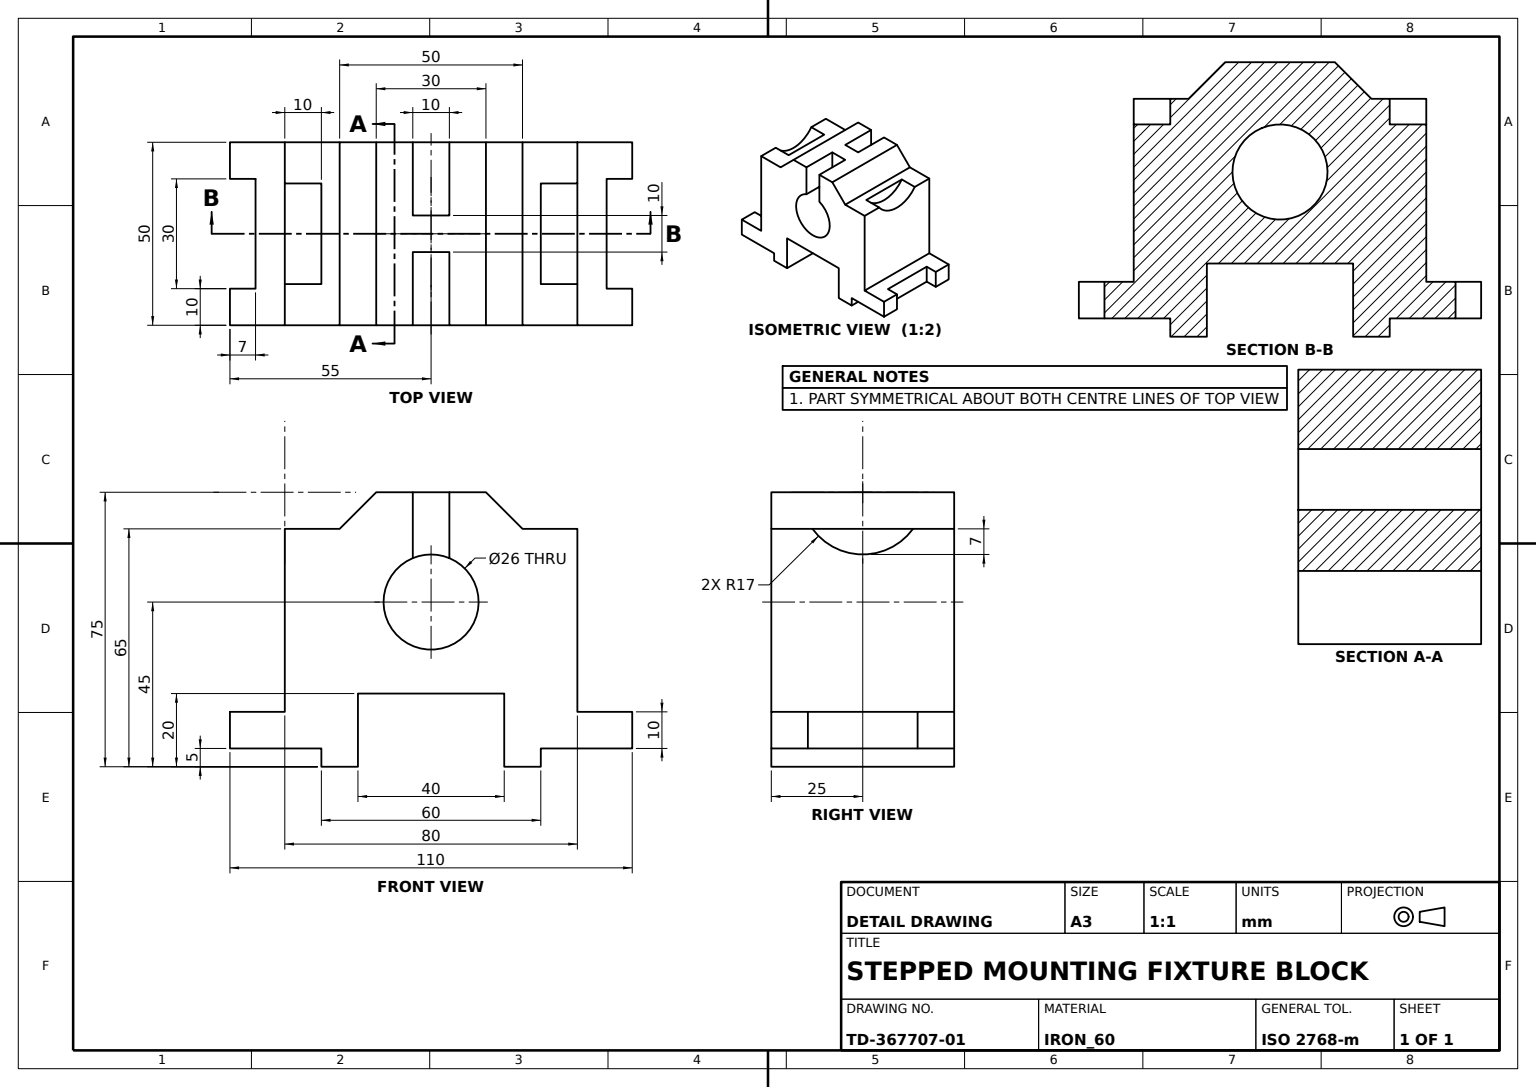
ISO-10303-21;
HEADER;
FILE_DESCRIPTION((''),'2;1');
FILE_NAME('','',(''),(''),'','','');
FILE_SCHEMA(('AUTOMOTIVE_DESIGN'));
ENDSEC;
DATA;
#1=APPLICATION_CONTEXT('');
#2=PRODUCT_CONTEXT('',#1,'mechanical');
#3=PRODUCT('','','',(#2));
#4=PRODUCT_DEFINITION_FORMATION('','',#3);
#5=PRODUCT_DEFINITION_CONTEXT('',#1,'design');
#6=PRODUCT_DEFINITION('','',#4,#5);
#7=PRODUCT_DEFINITION_SHAPE('','',#6);
#8=(LENGTH_UNIT()NAMED_UNIT(*)SI_UNIT(.MILLI.,.METRE.));
#9=(NAMED_UNIT(*)PLANE_ANGLE_UNIT()SI_UNIT($,.RADIAN.));
#10=(NAMED_UNIT(*)SI_UNIT($,.STERADIAN.)SOLID_ANGLE_UNIT());
#11=UNCERTAINTY_MEASURE_WITH_UNIT(LENGTH_MEASURE(0.005),#8,'distance_accuracy_value','');
#12=(GEOMETRIC_REPRESENTATION_CONTEXT(3)GLOBAL_UNCERTAINTY_ASSIGNED_CONTEXT((#11))GLOBAL_UNIT_ASSIGNED_CONTEXT((#8,#9,#10))REPRESENTATION_CONTEXT('',''));
#13=CARTESIAN_POINT('',(13.747727,-30.,60.));
#14=VERTEX_POINT('',#13);
#15=CARTESIAN_POINT('',(-13.747727,-30.,60.));
#16=VERTEX_POINT('',#15);
#17=CARTESIAN_POINT('',(25.,-30.,60.));
#18=DIRECTION('',(-1.,0.,0.));
#19=VECTOR('',#18,1000.);
#20=LINE('',#17,#19);
#21=EDGE_CURVE('',#14,#16,#20,.T.);
#22=ORIENTED_EDGE('',*,*,#21,.T.);
#23=CARTESIAN_POINT('',(0.,-30.,70.));
#24=DIRECTION('',(0.,-1.,0.));
#25=DIRECTION('',(1.,0.,0.));
#26=AXIS2_PLACEMENT_3D('',#23,#24,#25);
#27=CIRCLE('',#26,17.);
#28=EDGE_CURVE('',#14,#16,#27,.F.);
#29=ORIENTED_EDGE('',*,*,#28,.F.);
#30=EDGE_LOOP('',(#22,#29));
#31=FACE_BOUND('',#30,.T.);
#32=DIRECTION('',(0.,0.,-1.));
#33=AXIS2_PLACEMENT_3D('',#23,#24,#32);
#34=PLANE('',#33);
#35=ADVANCED_FACE('',(#31),#34,.T.);
#36=CARTESIAN_POINT('',(-15.,-55.,10.));
#37=VERTEX_POINT('',#36);
#38=CARTESIAN_POINT('',(-15.,-48.,10.));
#39=VERTEX_POINT('',#38);
#40=DIRECTION('',(0.,1.,0.));
#41=VECTOR('',#40,1000.);
#42=LINE('',#36,#41);
#43=EDGE_CURVE('',#37,#39,#42,.T.);
#44=ORIENTED_EDGE('',*,*,#43,.T.);
#45=CARTESIAN_POINT('',(15.,-48.,10.));
#46=VERTEX_POINT('',#45);
#47=CARTESIAN_POINT('',(25.,-48.,10.));
#48=VECTOR('',#25,1000.);
#49=LINE('',#47,#48);
#50=EDGE_CURVE('',#39,#46,#49,.T.);
#51=ORIENTED_EDGE('',*,*,#50,.T.);
#52=CARTESIAN_POINT('',(15.,-55.,10.));
#53=VERTEX_POINT('',#52);
#54=VECTOR('',#24,1000.);
#55=LINE('',#52,#54);
#56=EDGE_CURVE('',#46,#53,#55,.T.);
#57=ORIENTED_EDGE('',*,*,#56,.T.);
#58=CARTESIAN_POINT('',(25.,-55.,10.));
#59=VERTEX_POINT('',#58);
#60=LINE('',#58,#19);
#61=EDGE_CURVE('',#59,#53,#60,.T.);
#62=ORIENTED_EDGE('',*,*,#61,.F.);
#63=CARTESIAN_POINT('',(25.,-40.,10.));
#64=VERTEX_POINT('',#63);
#65=LINE('',#58,#41);
#66=EDGE_CURVE('',#59,#64,#65,.T.);
#67=ORIENTED_EDGE('',*,*,#66,.T.);
#68=CARTESIAN_POINT('',(-25.,-40.,10.));
#69=VERTEX_POINT('',#68);
#70=LINE('',#63,#19);
#71=EDGE_CURVE('',#64,#69,#70,.T.);
#72=ORIENTED_EDGE('',*,*,#71,.T.);
#73=CARTESIAN_POINT('',(-25.,-55.,10.));
#74=VERTEX_POINT('',#73);
#75=LINE('',#73,#41);
#76=EDGE_CURVE('',#74,#69,#75,.T.);
#77=ORIENTED_EDGE('',*,*,#76,.F.);
#78=EDGE_CURVE('',#37,#74,#60,.T.);
#79=ORIENTED_EDGE('',*,*,#78,.F.);
#80=EDGE_LOOP('',(#44,#51,#57,#62,#67,#72,#77,#79));
#81=FACE_BOUND('',#80,.T.);
#82=DIRECTION('',(0.,0.,1.));
#83=AXIS2_PLACEMENT_3D('',#58,#82,#25);
#84=PLANE('',#83);
#85=ADVANCED_FACE('',(#81),#84,.T.);
#86=CARTESIAN_POINT('',(25.,-40.,60.));
#87=VERTEX_POINT('',#86);
#88=CARTESIAN_POINT('',(13.747727,-40.,60.));
#89=VERTEX_POINT('',#88);
#90=LINE('',#86,#19);
#91=EDGE_CURVE('',#87,#89,#90,.T.);
#92=ORIENTED_EDGE('',*,*,#91,.F.);
#93=CARTESIAN_POINT('',(25.,-25.,60.));
#94=VERTEX_POINT('',#93);
#95=CARTESIAN_POINT('',(25.,40.,60.));
#96=LINE('',#95,#54);
#97=EDGE_CURVE('',#94,#87,#96,.T.);
#98=ORIENTED_EDGE('',*,*,#97,.F.);
#99=CARTESIAN_POINT('',(-25.,-25.,60.));
#100=VERTEX_POINT('',#99);
#101=LINE('',#93,#19);
#102=EDGE_CURVE('',#94,#100,#101,.T.);
#103=ORIENTED_EDGE('',*,*,#102,.T.);
#104=CARTESIAN_POINT('',(-25.,-40.,60.));
#105=VERTEX_POINT('',#104);
#106=CARTESIAN_POINT('',(-25.,40.,60.));
#107=LINE('',#106,#54);
#108=EDGE_CURVE('',#100,#105,#107,.T.);
#109=ORIENTED_EDGE('',*,*,#108,.T.);
#110=CARTESIAN_POINT('',(-13.747727,-40.,60.));
#111=VERTEX_POINT('',#110);
#112=EDGE_CURVE('',#111,#105,#90,.T.);
#113=ORIENTED_EDGE('',*,*,#112,.F.);
#114=CARTESIAN_POINT('',(-13.747727,-45.,60.));
#115=LINE('',#114,#41);
#116=EDGE_CURVE('',#16,#111,#115,.F.);
#117=ORIENTED_EDGE('',*,*,#116,.F.);
#118=ORIENTED_EDGE('',*,*,#21,.F.);
#119=CARTESIAN_POINT('',(13.747727,-45.,60.));
#120=LINE('',#119,#41);
#121=EDGE_CURVE('',#89,#14,#120,.T.);
#122=ORIENTED_EDGE('',*,*,#121,.F.);
#123=EDGE_LOOP('',(#92,#98,#103,#109,#113,#117,#118,#122));
#124=FACE_BOUND('',#123,.T.);
#125=AXIS2_PLACEMENT_3D('',#95,#32,#18);
#126=PLANE('',#125);
#127=ADVANCED_FACE('',(#124),#126,.F.);
#128=CARTESIAN_POINT('',(25.,5.,70.));
#129=VERTEX_POINT('',#128);
#130=CARTESIAN_POINT('',(5.,5.,70.));
#131=VERTEX_POINT('',#130);
#132=LINE('',#128,#19);
#133=EDGE_CURVE('',#129,#131,#132,.T.);
#134=ORIENTED_EDGE('',*,*,#133,.F.);
#135=CARTESIAN_POINT('',(25.,15.,70.));
#136=VERTEX_POINT('',#135);
#137=LINE('',#135,#54);
#138=EDGE_CURVE('',#136,#129,#137,.T.);
#139=ORIENTED_EDGE('',*,*,#138,.F.);
#140=CARTESIAN_POINT('',(-25.,15.,70.));
#141=VERTEX_POINT('',#140);
#142=LINE('',#135,#19);
#143=EDGE_CURVE('',#136,#141,#142,.T.);
#144=ORIENTED_EDGE('',*,*,#143,.T.);
#145=CARTESIAN_POINT('',(-25.,5.,70.));
#146=VERTEX_POINT('',#145);
#147=LINE('',#140,#54);
#148=EDGE_CURVE('',#141,#146,#147,.T.);
#149=ORIENTED_EDGE('',*,*,#148,.T.);
#150=CARTESIAN_POINT('',(-5.,5.,70.));
#151=VERTEX_POINT('',#150);
#152=LINE('',#128,#48);
#153=EDGE_CURVE('',#146,#151,#152,.T.);
#154=ORIENTED_EDGE('',*,*,#153,.T.);
#155=CARTESIAN_POINT('',(-5.,-5.,70.));
#156=VERTEX_POINT('',#155);
#157=CARTESIAN_POINT('',(-5.,15.,70.));
#158=LINE('',#157,#54);
#159=EDGE_CURVE('',#151,#156,#158,.T.);
#160=ORIENTED_EDGE('',*,*,#159,.T.);
#161=CARTESIAN_POINT('',(-25.,-5.,70.));
#162=VERTEX_POINT('',#161);
#163=CARTESIAN_POINT('',(25.,-5.,70.));
#164=LINE('',#163,#19);
#165=EDGE_CURVE('',#156,#162,#164,.T.);
#166=ORIENTED_EDGE('',*,*,#165,.T.);
#167=CARTESIAN_POINT('',(-25.,-15.,70.));
#168=VERTEX_POINT('',#167);
#169=EDGE_CURVE('',#162,#168,#147,.T.);
#170=ORIENTED_EDGE('',*,*,#169,.T.);
#171=CARTESIAN_POINT('',(25.,-15.,70.));
#172=VERTEX_POINT('',#171);
#173=LINE('',#171,#19);
#174=EDGE_CURVE('',#172,#168,#173,.T.);
#175=ORIENTED_EDGE('',*,*,#174,.F.);
#176=VERTEX_POINT('',#163);
#177=EDGE_CURVE('',#176,#172,#137,.T.);
#178=ORIENTED_EDGE('',*,*,#177,.F.);
#179=CARTESIAN_POINT('',(5.,-5.,70.));
#180=VERTEX_POINT('',#179);
#181=LINE('',#163,#48);
#182=EDGE_CURVE('',#180,#176,#181,.T.);
#183=ORIENTED_EDGE('',*,*,#182,.F.);
#184=CARTESIAN_POINT('',(5.,15.,70.));
#185=LINE('',#184,#54);
#186=EDGE_CURVE('',#131,#180,#185,.T.);
#187=ORIENTED_EDGE('',*,*,#186,.F.);
#188=EDGE_LOOP('',(#134,#139,#144,#149,#154,#160,#166,#170,#175,#178,#183,#187));
#189=FACE_BOUND('',#188,.T.);
#190=AXIS2_PLACEMENT_3D('',#135,#32,#18);
#191=PLANE('',#190);
#192=ADVANCED_FACE('',(#189),#191,.F.);
#193=CARTESIAN_POINT('',(25.,-55.,0.));
#194=VERTEX_POINT('',#193);
#195=CARTESIAN_POINT('',(15.,-55.,0.));
#196=VERTEX_POINT('',#195);
#197=LINE('',#193,#19);
#198=EDGE_CURVE('',#194,#196,#197,.T.);
#199=ORIENTED_EDGE('',*,*,#198,.T.);
#200=CARTESIAN_POINT('',(15.,-48.,0.));
#201=VERTEX_POINT('',#200);
#202=CARTESIAN_POINT('',(15.,55.,0.));
#203=LINE('',#202,#41);
#204=EDGE_CURVE('',#196,#201,#203,.T.);
#205=ORIENTED_EDGE('',*,*,#204,.T.);
#206=CARTESIAN_POINT('',(-15.,-48.,0.));
#207=VERTEX_POINT('',#206);
#208=CARTESIAN_POINT('',(25.,-48.,0.));
#209=LINE('',#208,#19);
#210=EDGE_CURVE('',#201,#207,#209,.T.);
#211=ORIENTED_EDGE('',*,*,#210,.T.);
#212=CARTESIAN_POINT('',(-15.,-55.,0.));
#213=VERTEX_POINT('',#212);
#214=CARTESIAN_POINT('',(-15.,55.,0.));
#215=LINE('',#214,#54);
#216=EDGE_CURVE('',#207,#213,#215,.T.);
#217=ORIENTED_EDGE('',*,*,#216,.T.);
#218=CARTESIAN_POINT('',(-25.,-55.,0.));
#219=VERTEX_POINT('',#218);
#220=EDGE_CURVE('',#213,#219,#197,.T.);
#221=ORIENTED_EDGE('',*,*,#220,.T.);
#222=CARTESIAN_POINT('',(-25.,-30.,0.));
#223=VERTEX_POINT('',#222);
#224=CARTESIAN_POINT('',(-25.,55.,0.));
#225=LINE('',#224,#54);
#226=EDGE_CURVE('',#223,#219,#225,.T.);
#227=ORIENTED_EDGE('',*,*,#226,.F.);
#228=CARTESIAN_POINT('',(25.,-30.,0.));
#229=VERTEX_POINT('',#228);
#230=LINE('',#228,#19);
#231=EDGE_CURVE('',#229,#223,#230,.T.);
#232=ORIENTED_EDGE('',*,*,#231,.F.);
#233=CARTESIAN_POINT('',(25.,55.,0.));
#234=LINE('',#233,#54);
#235=EDGE_CURVE('',#229,#194,#234,.T.);
#236=ORIENTED_EDGE('',*,*,#235,.T.);
#237=EDGE_LOOP('',(#199,#205,#211,#217,#221,#227,#232,#236));
#238=FACE_BOUND('',#237,.T.);
#239=AXIS2_PLACEMENT_3D('',#233,#32,#18);
#240=PLANE('',#239);
#241=ADVANCED_FACE('',(#238),#240,.T.);
#242=ORIENTED_EDGE('',*,*,#71,.F.);
#243=VECTOR('',#32,1000.);
#244=LINE('',#86,#243);
#245=EDGE_CURVE('',#87,#64,#244,.T.);
#246=ORIENTED_EDGE('',*,*,#245,.F.);
#247=ORIENTED_EDGE('',*,*,#91,.T.);
#248=CARTESIAN_POINT('',(0.,-40.,70.));
#249=AXIS2_PLACEMENT_3D('',#248,#40,#82);
#250=CIRCLE('',#249,17.);
#251=EDGE_CURVE('',#111,#89,#250,.F.);
#252=ORIENTED_EDGE('',*,*,#251,.F.);
#253=ORIENTED_EDGE('',*,*,#112,.T.);
#254=LINE('',#104,#243);
#255=EDGE_CURVE('',#105,#69,#254,.T.);
#256=ORIENTED_EDGE('',*,*,#255,.T.);
#257=EDGE_LOOP('',(#242,#246,#247,#252,#253,#256));
#258=FACE_BOUND('',#257,.T.);
#259=AXIS2_PLACEMENT_3D('',#86,#40,#82);
#260=PLANE('',#259);
#261=ADVANCED_FACE('',(#258),#260,.F.);
#262=VERTEX_POINT('',#106);
#263=CARTESIAN_POINT('',(-25.,25.,60.));
#264=VERTEX_POINT('',#263);
#265=EDGE_CURVE('',#262,#264,#107,.T.);
#266=ORIENTED_EDGE('',*,*,#265,.T.);
#267=CARTESIAN_POINT('',(25.,25.,60.));
#268=VERTEX_POINT('',#267);
#269=LINE('',#267,#19);
#270=EDGE_CURVE('',#268,#264,#269,.T.);
#271=ORIENTED_EDGE('',*,*,#270,.F.);
#272=VERTEX_POINT('',#95);
#273=EDGE_CURVE('',#272,#268,#96,.T.);
#274=ORIENTED_EDGE('',*,*,#273,.F.);
#275=CARTESIAN_POINT('',(13.747727,40.,60.));
#276=VERTEX_POINT('',#275);
#277=LINE('',#95,#19);
#278=EDGE_CURVE('',#272,#276,#277,.T.);
#279=ORIENTED_EDGE('',*,*,#278,.T.);
#280=CARTESIAN_POINT('',(13.747727,30.,60.));
#281=VERTEX_POINT('',#280);
#282=CARTESIAN_POINT('',(13.747727,45.,60.));
#283=LINE('',#282,#54);
#284=EDGE_CURVE('',#276,#281,#283,.T.);
#285=ORIENTED_EDGE('',*,*,#284,.T.);
#286=CARTESIAN_POINT('',(-13.747727,30.,60.));
#287=VERTEX_POINT('',#286);
#288=CARTESIAN_POINT('',(25.,30.,60.));
#289=LINE('',#288,#19);
#290=EDGE_CURVE('',#281,#287,#289,.T.);
#291=ORIENTED_EDGE('',*,*,#290,.T.);
#292=CARTESIAN_POINT('',(-13.747727,40.,60.));
#293=VERTEX_POINT('',#292);
#294=CARTESIAN_POINT('',(-13.747727,45.,60.));
#295=LINE('',#294,#54);
#296=EDGE_CURVE('',#287,#293,#295,.F.);
#297=ORIENTED_EDGE('',*,*,#296,.T.);
#298=EDGE_CURVE('',#293,#262,#277,.T.);
#299=ORIENTED_EDGE('',*,*,#298,.T.);
#300=EDGE_LOOP('',(#266,#271,#274,#279,#285,#291,#297,#299));
#301=FACE_BOUND('',#300,.T.);
#302=ADVANCED_FACE('',(#301),#126,.F.);
#303=ORIENTED_EDGE('',*,*,#198,.F.);
#304=VECTOR('',#82,1000.);
#305=LINE('',#193,#304);
#306=EDGE_CURVE('',#194,#59,#305,.T.);
#307=ORIENTED_EDGE('',*,*,#306,.T.);
#308=ORIENTED_EDGE('',*,*,#61,.T.);
#309=LINE('',#195,#243);
#310=EDGE_CURVE('',#53,#196,#309,.T.);
#311=ORIENTED_EDGE('',*,*,#310,.T.);
#312=EDGE_LOOP('',(#303,#307,#308,#311));
#313=FACE_BOUND('',#312,.T.);
#314=AXIS2_PLACEMENT_3D('',#193,#24,#32);
#315=PLANE('',#314);
#316=ADVANCED_FACE('',(#313),#315,.T.);
#317=CARTESIAN_POINT('',(-5.,-5.,52.));
#318=VERTEX_POINT('',#317);
#319=CARTESIAN_POINT('',(-5.,-5.,78.));
#320=LINE('',#319,#243);
#321=EDGE_CURVE('',#318,#156,#320,.F.);
#322=ORIENTED_EDGE('',*,*,#321,.F.);
#323=CARTESIAN_POINT('',(-25.,-5.,52.));
#324=VERTEX_POINT('',#323);
#325=CARTESIAN_POINT('',(25.,-5.,52.));
#326=LINE('',#325,#19);
#327=EDGE_CURVE('',#324,#318,#326,.F.);
#328=ORIENTED_EDGE('',*,*,#327,.F.);
#329=CARTESIAN_POINT('',(-25.,-5.,78.));
#330=LINE('',#329,#243);
#331=EDGE_CURVE('',#324,#162,#330,.F.);
#332=ORIENTED_EDGE('',*,*,#331,.T.);
#333=ORIENTED_EDGE('',*,*,#165,.F.);
#334=EDGE_LOOP('',(#322,#328,#332,#333));
#335=FACE_BOUND('',#334,.T.);
#336=AXIS2_PLACEMENT_3D('',#319,#24,#25);
#337=PLANE('',#336);
#338=ADVANCED_FACE('',(#335),#337,.F.);
#339=ORIENTED_EDGE('',*,*,#116,.T.);
#340=ORIENTED_EDGE('',*,*,#251,.T.);
#341=ORIENTED_EDGE('',*,*,#121,.T.);
#342=ORIENTED_EDGE('',*,*,#28,.T.);
#343=EDGE_LOOP('',(#339,#340,#341,#342));
#344=FACE_BOUND('',#343,.T.);
#345=CARTESIAN_POINT('',(0.,-45.,70.));
#346=AXIS2_PLACEMENT_3D('',#345,#40,#82);
#347=CYLINDRICAL_SURFACE('',#346,17.);
#348=ADVANCED_FACE('',(#344),#347,.F.);
#349=CARTESIAN_POINT('',(15.,48.,10.));
#350=VERTEX_POINT('',#349);
#351=CARTESIAN_POINT('',(15.,55.,10.));
#352=VERTEX_POINT('',#351);
#353=LINE('',#52,#41);
#354=EDGE_CURVE('',#350,#352,#353,.T.);
#355=ORIENTED_EDGE('',*,*,#354,.T.);
#356=VERTEX_POINT('',#202);
#357=LINE('',#351,#243);
#358=EDGE_CURVE('',#352,#356,#357,.T.);
#359=ORIENTED_EDGE('',*,*,#358,.T.);
#360=CARTESIAN_POINT('',(15.,48.,0.));
#361=VERTEX_POINT('',#360);
#362=LINE('',#202,#54);
#363=EDGE_CURVE('',#356,#361,#362,.T.);
#364=ORIENTED_EDGE('',*,*,#363,.T.);
#365=CARTESIAN_POINT('',(15.,48.,45.));
#366=LINE('',#365,#243);
#367=EDGE_CURVE('',#361,#350,#366,.F.);
#368=ORIENTED_EDGE('',*,*,#367,.T.);
#369=EDGE_LOOP('',(#355,#359,#364,#368));
#370=FACE_BOUND('',#369,.T.);
#371=CARTESIAN_POINT('',(15.,68.,45.));
#372=AXIS2_PLACEMENT_3D('',#371,#25,#40);
#373=PLANE('',#372);
#374=ADVANCED_FACE('',(#370),#373,.F.);
#375=CARTESIAN_POINT('',(25.,30.,-5.));
#376=VERTEX_POINT('',#375);
#377=CARTESIAN_POINT('',(-25.,30.,-5.));
#378=VERTEX_POINT('',#377);
#379=LINE('',#375,#19);
#380=EDGE_CURVE('',#376,#378,#379,.T.);
#381=ORIENTED_EDGE('',*,*,#380,.F.);
#382=CARTESIAN_POINT('',(25.,20.,-5.));
#383=VERTEX_POINT('',#382);
#384=LINE('',#382,#41);
#385=EDGE_CURVE('',#383,#376,#384,.T.);
#386=ORIENTED_EDGE('',*,*,#385,.F.);
#387=CARTESIAN_POINT('',(-25.,20.,-5.));
#388=VERTEX_POINT('',#387);
#389=LINE('',#382,#19);
#390=EDGE_CURVE('',#383,#388,#389,.T.);
#391=ORIENTED_EDGE('',*,*,#390,.T.);
#392=LINE('',#387,#41);
#393=EDGE_CURVE('',#388,#378,#392,.T.);
#394=ORIENTED_EDGE('',*,*,#393,.T.);
#395=EDGE_LOOP('',(#381,#386,#391,#394));
#396=FACE_BOUND('',#395,.T.);
#397=AXIS2_PLACEMENT_3D('',#382,#82,#24);
#398=PLANE('',#397);
#399=ADVANCED_FACE('',(#396),#398,.F.);
#400=VERTEX_POINT('',#224);
#401=CARTESIAN_POINT('',(-25.,30.,0.));
#402=VERTEX_POINT('',#401);
#403=EDGE_CURVE('',#400,#402,#225,.T.);
#404=ORIENTED_EDGE('',*,*,#403,.T.);
#405=LINE('',#377,#304);
#406=EDGE_CURVE('',#378,#402,#405,.T.);
#407=ORIENTED_EDGE('',*,*,#406,.F.);
#408=ORIENTED_EDGE('',*,*,#393,.F.);
#409=CARTESIAN_POINT('',(-25.,20.,15.));
#410=VERTEX_POINT('',#409);
#411=CARTESIAN_POINT('',(-25.,20.,0.));
#412=LINE('',#411,#243);
#413=EDGE_CURVE('',#410,#388,#412,.T.);
#414=ORIENTED_EDGE('',*,*,#413,.F.);
#415=CARTESIAN_POINT('',(-25.,-20.,15.));
#416=VERTEX_POINT('',#415);
#417=CARTESIAN_POINT('',(-25.,0.,15.));
#418=LINE('',#417,#41);
#419=EDGE_CURVE('',#416,#410,#418,.T.);
#420=ORIENTED_EDGE('',*,*,#419,.F.);
#421=CARTESIAN_POINT('',(-25.,-20.,-5.));
#422=VERTEX_POINT('',#421);
#423=CARTESIAN_POINT('',(-25.,-20.,0.));
#424=LINE('',#423,#243);
#425=EDGE_CURVE('',#416,#422,#424,.T.);
#426=ORIENTED_EDGE('',*,*,#425,.T.);
#427=CARTESIAN_POINT('',(-25.,-30.,-5.));
#428=VERTEX_POINT('',#427);
#429=LINE('',#421,#54);
#430=EDGE_CURVE('',#422,#428,#429,.T.);
#431=ORIENTED_EDGE('',*,*,#430,.T.);
#432=LINE('',#427,#304);
#433=EDGE_CURVE('',#428,#223,#432,.T.);
#434=ORIENTED_EDGE('',*,*,#433,.T.);
#435=ORIENTED_EDGE('',*,*,#226,.T.);
#436=LINE('',#218,#304);
#437=EDGE_CURVE('',#219,#74,#436,.T.);
#438=ORIENTED_EDGE('',*,*,#437,.T.);
#439=ORIENTED_EDGE('',*,*,#76,.T.);
#440=ORIENTED_EDGE('',*,*,#255,.F.);
#441=ORIENTED_EDGE('',*,*,#108,.F.);
#442=DIRECTION('',(0.,-0.707106781,-0.707106781));
#443=VECTOR('',#442,1000.);
#444=LINE('',#167,#443);
#445=EDGE_CURVE('',#168,#100,#444,.T.);
#446=ORIENTED_EDGE('',*,*,#445,.F.);
#447=ORIENTED_EDGE('',*,*,#169,.F.);
#448=ORIENTED_EDGE('',*,*,#331,.F.);
#449=CARTESIAN_POINT('',(-25.,5.,52.));
#450=VERTEX_POINT('',#449);
#451=CARTESIAN_POINT('',(-25.,0.,40.));
#452=AXIS2_PLACEMENT_3D('',#451,#18,#82);
#453=CIRCLE('',#452,13.);
#454=EDGE_CURVE('',#450,#324,#453,.T.);
#455=ORIENTED_EDGE('',*,*,#454,.F.);
#456=CARTESIAN_POINT('',(-25.,5.,78.));
#457=LINE('',#456,#243);
#458=EDGE_CURVE('',#146,#450,#457,.T.);
#459=ORIENTED_EDGE('',*,*,#458,.F.);
#460=ORIENTED_EDGE('',*,*,#148,.F.);
#461=DIRECTION('',(0.,-0.707106781,0.707106781));
#462=VECTOR('',#461,1000.);
#463=LINE('',#263,#462);
#464=EDGE_CURVE('',#264,#141,#463,.T.);
#465=ORIENTED_EDGE('',*,*,#464,.F.);
#466=ORIENTED_EDGE('',*,*,#265,.F.);
#467=CARTESIAN_POINT('',(-25.,40.,10.));
#468=VERTEX_POINT('',#467);
#469=LINE('',#467,#304);
#470=EDGE_CURVE('',#468,#262,#469,.T.);
#471=ORIENTED_EDGE('',*,*,#470,.F.);
#472=CARTESIAN_POINT('',(-25.,55.,10.));
#473=VERTEX_POINT('',#472);
#474=EDGE_CURVE('',#468,#473,#75,.T.);
#475=ORIENTED_EDGE('',*,*,#474,.T.);
#476=LINE('',#472,#243);
#477=EDGE_CURVE('',#473,#400,#476,.T.);
#478=ORIENTED_EDGE('',*,*,#477,.T.);
#479=EDGE_LOOP('',(#404,#407,#408,#414,#420,#426,#431,#434,#435,#438,#439,#440,#441,#446,#447,#448,#455,#459,#460,#465,#466,#471,#475,#478));
#480=FACE_BOUND('',#479,.T.);
#481=CARTESIAN_POINT('',(-25.,0.,0.));
#482=AXIS2_PLACEMENT_3D('',#481,#18,#82);
#483=PLANE('',#482);
#484=ADVANCED_FACE('',(#480),#483,.T.);
#485=CARTESIAN_POINT('',(-15.,-48.,45.));
#486=LINE('',#485,#243);
#487=EDGE_CURVE('',#207,#39,#486,.F.);
#488=ORIENTED_EDGE('',*,*,#487,.T.);
#489=ORIENTED_EDGE('',*,*,#43,.F.);
#490=LINE('',#212,#304);
#491=EDGE_CURVE('',#213,#37,#490,.T.);
#492=ORIENTED_EDGE('',*,*,#491,.F.);
#493=ORIENTED_EDGE('',*,*,#216,.F.);
#494=EDGE_LOOP('',(#488,#489,#492,#493));
#495=FACE_BOUND('',#494,.T.);
#496=AXIS2_PLACEMENT_3D('',#485,#25,#40);
#497=PLANE('',#496);
#498=ADVANCED_FACE('',(#495),#497,.T.);
#499=ORIENTED_EDGE('',*,*,#419,.T.);
#500=CARTESIAN_POINT('',(25.,20.,15.));
#501=VERTEX_POINT('',#500);
#502=CARTESIAN_POINT('',(26.,20.,15.));
#503=LINE('',#502,#19);
#504=EDGE_CURVE('',#501,#410,#503,.T.);
#505=ORIENTED_EDGE('',*,*,#504,.F.);
#506=CARTESIAN_POINT('',(25.,-20.,15.));
#507=VERTEX_POINT('',#506);
#508=CARTESIAN_POINT('',(25.,0.,15.));
#509=LINE('',#508,#41);
#510=EDGE_CURVE('',#507,#501,#509,.T.);
#511=ORIENTED_EDGE('',*,*,#510,.F.);
#512=CARTESIAN_POINT('',(26.,-20.,15.));
#513=LINE('',#512,#19);
#514=EDGE_CURVE('',#507,#416,#513,.T.);
#515=ORIENTED_EDGE('',*,*,#514,.T.);
#516=EDGE_LOOP('',(#499,#505,#511,#515));
#517=FACE_BOUND('',#516,.T.);
#518=AXIS2_PLACEMENT_3D('',#512,#82,#25);
#519=PLANE('',#518);
#520=ADVANCED_FACE('',(#517),#519,.F.);
#521=CARTESIAN_POINT('',(25.,-30.,-5.));
#522=VERTEX_POINT('',#521);
#523=LINE('',#521,#304);
#524=EDGE_CURVE('',#522,#229,#523,.T.);
#525=ORIENTED_EDGE('',*,*,#524,.T.);
#526=ORIENTED_EDGE('',*,*,#231,.T.);
#527=ORIENTED_EDGE('',*,*,#433,.F.);
#528=LINE('',#521,#19);
#529=EDGE_CURVE('',#522,#428,#528,.T.);
#530=ORIENTED_EDGE('',*,*,#529,.F.);
#531=EDGE_LOOP('',(#525,#526,#527,#530));
#532=FACE_BOUND('',#531,.T.);
#533=AXIS2_PLACEMENT_3D('',#521,#24,#32);
#534=PLANE('',#533);
#535=ADVANCED_FACE('',(#532),#534,.T.);
#536=ORIENTED_EDGE('',*,*,#358,.F.);
#537=CARTESIAN_POINT('',(25.,55.,10.));
#538=VERTEX_POINT('',#537);
#539=LINE('',#537,#19);
#540=EDGE_CURVE('',#538,#352,#539,.T.);
#541=ORIENTED_EDGE('',*,*,#540,.F.);
#542=VERTEX_POINT('',#233);
#543=LINE('',#537,#243);
#544=EDGE_CURVE('',#538,#542,#543,.T.);
#545=ORIENTED_EDGE('',*,*,#544,.T.);
#546=LINE('',#233,#19);
#547=EDGE_CURVE('',#542,#356,#546,.T.);
#548=ORIENTED_EDGE('',*,*,#547,.T.);
#549=EDGE_LOOP('',(#536,#541,#545,#548));
#550=FACE_BOUND('',#549,.T.);
#551=AXIS2_PLACEMENT_3D('',#537,#40,#82);
#552=PLANE('',#551);
#553=ADVANCED_FACE('',(#550),#552,.T.);
#554=ORIENTED_EDGE('',*,*,#186,.T.);
#555=CARTESIAN_POINT('',(5.,-5.,52.));
#556=VERTEX_POINT('',#555);
#557=CARTESIAN_POINT('',(5.,-5.,78.));
#558=LINE('',#557,#243);
#559=EDGE_CURVE('',#556,#180,#558,.F.);
#560=ORIENTED_EDGE('',*,*,#559,.F.);
#561=CARTESIAN_POINT('',(5.,5.,52.));
#562=VERTEX_POINT('',#561);
#563=CARTESIAN_POINT('',(5.,0.,40.));
#564=AXIS2_PLACEMENT_3D('',#563,#25,#32);
#565=CIRCLE('',#564,13.);
#566=EDGE_CURVE('',#556,#562,#565,.F.);
#567=ORIENTED_EDGE('',*,*,#566,.T.);
#568=CARTESIAN_POINT('',(5.,5.,78.));
#569=LINE('',#568,#243);
#570=EDGE_CURVE('',#562,#131,#569,.F.);
#571=ORIENTED_EDGE('',*,*,#570,.T.);
#572=EDGE_LOOP('',(#554,#560,#567,#571));
#573=FACE_BOUND('',#572,.T.);
#574=AXIS2_PLACEMENT_3D('',#568,#25,#32);
#575=PLANE('',#574);
#576=ADVANCED_FACE('',(#573),#575,.T.);
#577=ORIENTED_EDGE('',*,*,#406,.T.);
#578=CARTESIAN_POINT('',(25.,30.,0.));
#579=VERTEX_POINT('',#578);
#580=LINE('',#578,#19);
#581=EDGE_CURVE('',#579,#402,#580,.T.);
#582=ORIENTED_EDGE('',*,*,#581,.F.);
#583=LINE('',#375,#304);
#584=EDGE_CURVE('',#376,#579,#583,.T.);
#585=ORIENTED_EDGE('',*,*,#584,.F.);
#586=ORIENTED_EDGE('',*,*,#380,.T.);
#587=EDGE_LOOP('',(#577,#582,#585,#586));
#588=FACE_BOUND('',#587,.T.);
#589=AXIS2_PLACEMENT_3D('',#375,#24,#32);
#590=PLANE('',#589);
#591=ADVANCED_FACE('',(#588),#590,.F.);
#592=CARTESIAN_POINT('',(-15.,48.,0.));
#593=VERTEX_POINT('',#592);
#594=CARTESIAN_POINT('',(-15.,48.,10.));
#595=VERTEX_POINT('',#594);
#596=CARTESIAN_POINT('',(-15.,48.,45.));
#597=LINE('',#596,#243);
#598=EDGE_CURVE('',#593,#595,#597,.F.);
#599=ORIENTED_EDGE('',*,*,#598,.F.);
#600=VERTEX_POINT('',#214);
#601=LINE('',#214,#41);
#602=EDGE_CURVE('',#593,#600,#601,.T.);
#603=ORIENTED_EDGE('',*,*,#602,.T.);
#604=CARTESIAN_POINT('',(-15.,55.,10.));
#605=VERTEX_POINT('',#604);
#606=LINE('',#604,#304);
#607=EDGE_CURVE('',#600,#605,#606,.T.);
#608=ORIENTED_EDGE('',*,*,#607,.T.);
#609=LINE('',#36,#54);
#610=EDGE_CURVE('',#605,#595,#609,.T.);
#611=ORIENTED_EDGE('',*,*,#610,.T.);
#612=EDGE_LOOP('',(#599,#603,#608,#611));
#613=FACE_BOUND('',#612,.T.);
#614=AXIS2_PLACEMENT_3D('',#596,#18,#24);
#615=PLANE('',#614);
#616=ADVANCED_FACE('',(#613),#615,.F.);
#617=ORIENTED_EDGE('',*,*,#153,.F.);
#618=ORIENTED_EDGE('',*,*,#458,.T.);
#619=CARTESIAN_POINT('',(-5.,5.,52.));
#620=VERTEX_POINT('',#619);
#621=CARTESIAN_POINT('',(25.,5.,52.));
#622=LINE('',#621,#19);
#623=EDGE_CURVE('',#620,#450,#622,.T.);
#624=ORIENTED_EDGE('',*,*,#623,.F.);
#625=CARTESIAN_POINT('',(-5.,5.,78.));
#626=LINE('',#625,#243);
#627=EDGE_CURVE('',#620,#151,#626,.F.);
#628=ORIENTED_EDGE('',*,*,#627,.T.);
#629=EDGE_LOOP('',(#617,#618,#624,#628));
#630=FACE_BOUND('',#629,.T.);
#631=AXIS2_PLACEMENT_3D('',#456,#40,#18);
#632=PLANE('',#631);
#633=ADVANCED_FACE('',(#630),#632,.F.);
#634=ORIENTED_EDGE('',*,*,#133,.T.);
#635=ORIENTED_EDGE('',*,*,#570,.F.);
#636=VERTEX_POINT('',#621);
#637=EDGE_CURVE('',#562,#636,#622,.F.);
#638=ORIENTED_EDGE('',*,*,#637,.T.);
#639=CARTESIAN_POINT('',(25.,5.,78.));
#640=LINE('',#639,#243);
#641=EDGE_CURVE('',#636,#129,#640,.F.);
#642=ORIENTED_EDGE('',*,*,#641,.T.);
#643=EDGE_LOOP('',(#634,#635,#638,#642));
#644=FACE_BOUND('',#643,.T.);
#645=AXIS2_PLACEMENT_3D('',#639,#24,#25);
#646=PLANE('',#645);
#647=ADVANCED_FACE('',(#644),#646,.T.);
#648=LINE('',#171,#443);
#649=EDGE_CURVE('',#172,#94,#648,.T.);
#650=ORIENTED_EDGE('',*,*,#649,.F.);
#651=ORIENTED_EDGE('',*,*,#174,.T.);
#652=ORIENTED_EDGE('',*,*,#445,.T.);
#653=ORIENTED_EDGE('',*,*,#102,.F.);
#654=EDGE_LOOP('',(#650,#651,#652,#653));
#655=FACE_BOUND('',#654,.T.);
#656=DIRECTION('',(0.,0.707106781,-0.707106781));
#657=DIRECTION('',(0.,0.707106781,0.707106781));
#658=AXIS2_PLACEMENT_3D('',#171,#656,#657);
#659=PLANE('',#658);
#660=ADVANCED_FACE('',(#655),#659,.F.);
#661=CARTESIAN_POINT('',(-5.,0.,40.));
#662=AXIS2_PLACEMENT_3D('',#661,#25,#32);
#663=CIRCLE('',#662,13.);
#664=EDGE_CURVE('',#318,#620,#663,.F.);
#665=ORIENTED_EDGE('',*,*,#664,.F.);
#666=ORIENTED_EDGE('',*,*,#321,.T.);
#667=ORIENTED_EDGE('',*,*,#159,.F.);
#668=ORIENTED_EDGE('',*,*,#627,.F.);
#669=EDGE_LOOP('',(#665,#666,#667,#668));
#670=FACE_BOUND('',#669,.T.);
#671=AXIS2_PLACEMENT_3D('',#625,#25,#32);
#672=PLANE('',#671);
#673=ADVANCED_FACE('',(#670),#672,.F.);
#674=ORIENTED_EDGE('',*,*,#559,.T.);
#675=ORIENTED_EDGE('',*,*,#182,.T.);
#676=VERTEX_POINT('',#325);
#677=CARTESIAN_POINT('',(25.,-5.,78.));
#678=LINE('',#677,#243);
#679=EDGE_CURVE('',#176,#676,#678,.T.);
#680=ORIENTED_EDGE('',*,*,#679,.T.);
#681=EDGE_CURVE('',#676,#556,#326,.T.);
#682=ORIENTED_EDGE('',*,*,#681,.T.);
#683=EDGE_LOOP('',(#674,#675,#680,#682));
#684=FACE_BOUND('',#683,.T.);
#685=AXIS2_PLACEMENT_3D('',#557,#40,#18);
#686=PLANE('',#685);
#687=ADVANCED_FACE('',(#684),#686,.T.);
#688=CARTESIAN_POINT('',(25.,40.,10.));
#689=VERTEX_POINT('',#688);
#690=LINE('',#688,#19);
#691=EDGE_CURVE('',#689,#468,#690,.T.);
#692=ORIENTED_EDGE('',*,*,#691,.F.);
#693=EDGE_CURVE('',#689,#538,#65,.T.);
#694=ORIENTED_EDGE('',*,*,#693,.T.);
#695=ORIENTED_EDGE('',*,*,#540,.T.);
#696=ORIENTED_EDGE('',*,*,#354,.F.);
#697=CARTESIAN_POINT('',(25.,48.,10.));
#698=LINE('',#697,#48);
#699=EDGE_CURVE('',#595,#350,#698,.T.);
#700=ORIENTED_EDGE('',*,*,#699,.F.);
#701=ORIENTED_EDGE('',*,*,#610,.F.);
#702=EDGE_CURVE('',#605,#473,#539,.T.);
#703=ORIENTED_EDGE('',*,*,#702,.T.);
#704=ORIENTED_EDGE('',*,*,#474,.F.);
#705=EDGE_LOOP('',(#692,#694,#695,#696,#700,#701,#703,#704));
#706=FACE_BOUND('',#705,.T.);
#707=ADVANCED_FACE('',(#706),#84,.T.);
#708=EDGE_CURVE('',#600,#400,#546,.T.);
#709=ORIENTED_EDGE('',*,*,#708,.T.);
#710=ORIENTED_EDGE('',*,*,#477,.F.);
#711=ORIENTED_EDGE('',*,*,#702,.F.);
#712=ORIENTED_EDGE('',*,*,#607,.F.);
#713=EDGE_LOOP('',(#709,#710,#711,#712));
#714=FACE_BOUND('',#713,.T.);
#715=ADVANCED_FACE('',(#714),#552,.T.);
#716=ORIENTED_EDGE('',*,*,#470,.T.);
#717=ORIENTED_EDGE('',*,*,#298,.F.);
#718=CARTESIAN_POINT('',(0.,40.,70.));
#719=AXIS2_PLACEMENT_3D('',#718,#24,#32);
#720=CIRCLE('',#719,17.);
#721=EDGE_CURVE('',#293,#276,#720,.T.);
#722=ORIENTED_EDGE('',*,*,#721,.T.);
#723=ORIENTED_EDGE('',*,*,#278,.F.);
#724=LINE('',#688,#304);
#725=EDGE_CURVE('',#689,#272,#724,.T.);
#726=ORIENTED_EDGE('',*,*,#725,.F.);
#727=ORIENTED_EDGE('',*,*,#691,.T.);
#728=EDGE_LOOP('',(#716,#717,#722,#723,#726,#727));
#729=FACE_BOUND('',#728,.T.);
#730=AXIS2_PLACEMENT_3D('',#688,#24,#32);
#731=PLANE('',#730);
#732=ADVANCED_FACE('',(#729),#731,.F.);
#733=ORIENTED_EDGE('',*,*,#270,.T.);
#734=ORIENTED_EDGE('',*,*,#464,.T.);
#735=ORIENTED_EDGE('',*,*,#143,.F.);
#736=LINE('',#267,#462);
#737=EDGE_CURVE('',#268,#136,#736,.T.);
#738=ORIENTED_EDGE('',*,*,#737,.F.);
#739=EDGE_LOOP('',(#733,#734,#735,#738));
#740=FACE_BOUND('',#739,.T.);
#741=AXIS2_PLACEMENT_3D('',#267,#442,#656);
#742=PLANE('',#741);
#743=ADVANCED_FACE('',(#740),#742,.F.);
#744=ORIENTED_EDGE('',*,*,#504,.T.);
#745=ORIENTED_EDGE('',*,*,#413,.T.);
#746=ORIENTED_EDGE('',*,*,#390,.F.);
#747=CARTESIAN_POINT('',(25.,20.,0.));
#748=LINE('',#747,#243);
#749=EDGE_CURVE('',#501,#383,#748,.T.);
#750=ORIENTED_EDGE('',*,*,#749,.F.);
#751=EDGE_LOOP('',(#744,#745,#746,#750));
#752=FACE_BOUND('',#751,.T.);
#753=AXIS2_PLACEMENT_3D('',#747,#40,#82);
#754=PLANE('',#753);
#755=ADVANCED_FACE('',(#752),#754,.F.);
#756=ORIENTED_EDGE('',*,*,#425,.F.);
#757=ORIENTED_EDGE('',*,*,#514,.F.);
#758=CARTESIAN_POINT('',(25.,-20.,-5.));
#759=VERTEX_POINT('',#758);
#760=CARTESIAN_POINT('',(25.,-20.,0.));
#761=LINE('',#760,#243);
#762=EDGE_CURVE('',#507,#759,#761,.T.);
#763=ORIENTED_EDGE('',*,*,#762,.T.);
#764=LINE('',#758,#19);
#765=EDGE_CURVE('',#759,#422,#764,.T.);
#766=ORIENTED_EDGE('',*,*,#765,.T.);
#767=EDGE_LOOP('',(#756,#757,#763,#766));
#768=FACE_BOUND('',#767,.T.);
#769=AXIS2_PLACEMENT_3D('',#760,#40,#82);
#770=PLANE('',#769);
#771=ADVANCED_FACE('',(#768),#770,.T.);
#772=ORIENTED_EDGE('',*,*,#78,.T.);
#773=ORIENTED_EDGE('',*,*,#437,.F.);
#774=ORIENTED_EDGE('',*,*,#220,.F.);
#775=ORIENTED_EDGE('',*,*,#491,.T.);
#776=EDGE_LOOP('',(#772,#773,#774,#775));
#777=FACE_BOUND('',#776,.T.);
#778=ADVANCED_FACE('',(#777),#315,.T.);
#779=ORIENTED_EDGE('',*,*,#56,.F.);
#780=CARTESIAN_POINT('',(15.,-48.,45.));
#781=LINE('',#780,#243);
#782=EDGE_CURVE('',#201,#46,#781,.F.);
#783=ORIENTED_EDGE('',*,*,#782,.F.);
#784=ORIENTED_EDGE('',*,*,#204,.F.);
#785=ORIENTED_EDGE('',*,*,#310,.F.);
#786=EDGE_LOOP('',(#779,#783,#784,#785));
#787=FACE_BOUND('',#786,.T.);
#788=CARTESIAN_POINT('',(15.,-68.,45.));
#789=AXIS2_PLACEMENT_3D('',#788,#18,#24);
#790=PLANE('',#789);
#791=ADVANCED_FACE('',(#787),#790,.T.);
#792=ORIENTED_EDGE('',*,*,#721,.F.);
#793=ORIENTED_EDGE('',*,*,#296,.F.);
#794=CARTESIAN_POINT('',(0.,30.,70.));
#795=AXIS2_PLACEMENT_3D('',#794,#24,#25);
#796=CIRCLE('',#795,17.);
#797=EDGE_CURVE('',#281,#287,#796,.F.);
#798=ORIENTED_EDGE('',*,*,#797,.F.);
#799=ORIENTED_EDGE('',*,*,#284,.F.);
#800=EDGE_LOOP('',(#792,#793,#798,#799));
#801=FACE_BOUND('',#800,.T.);
#802=CARTESIAN_POINT('',(0.,45.,70.));
#803=AXIS2_PLACEMENT_3D('',#802,#24,#32);
#804=CYLINDRICAL_SURFACE('',#803,17.);
#805=ADVANCED_FACE('',(#801),#804,.F.);
#806=CARTESIAN_POINT('',(25.,48.,0.));
#807=LINE('',#806,#19);
#808=EDGE_CURVE('',#361,#593,#807,.T.);
#809=ORIENTED_EDGE('',*,*,#808,.T.);
#810=ORIENTED_EDGE('',*,*,#598,.T.);
#811=ORIENTED_EDGE('',*,*,#699,.T.);
#812=ORIENTED_EDGE('',*,*,#367,.F.);
#813=EDGE_LOOP('',(#809,#810,#811,#812));
#814=FACE_BOUND('',#813,.T.);
#815=AXIS2_PLACEMENT_3D('',#365,#24,#32);
#816=PLANE('',#815);
#817=ADVANCED_FACE('',(#814),#816,.F.);
#818=ORIENTED_EDGE('',*,*,#327,.T.);
#819=ORIENTED_EDGE('',*,*,#664,.T.);
#820=ORIENTED_EDGE('',*,*,#623,.T.);
#821=ORIENTED_EDGE('',*,*,#454,.T.);
#822=EDGE_LOOP('',(#818,#819,#820,#821));
#823=FACE_BOUND('',#822,.T.);
#824=ORIENTED_EDGE('',*,*,#637,.F.);
#825=ORIENTED_EDGE('',*,*,#566,.F.);
#826=ORIENTED_EDGE('',*,*,#681,.F.);
#827=CARTESIAN_POINT('',(25.,0.,40.));
#828=AXIS2_PLACEMENT_3D('',#827,#18,#82);
#829=CIRCLE('',#828,13.);
#830=EDGE_CURVE('',#636,#676,#829,.T.);
#831=ORIENTED_EDGE('',*,*,#830,.F.);
#832=EDGE_LOOP('',(#824,#825,#826,#831));
#833=FACE_BOUND('',#832,.T.);
#834=CYLINDRICAL_SURFACE('',#828,13.);
#835=ADVANCED_FACE('',(#823,#833),#834,.F.);
#836=ORIENTED_EDGE('',*,*,#487,.F.);
#837=ORIENTED_EDGE('',*,*,#210,.F.);
#838=ORIENTED_EDGE('',*,*,#782,.T.);
#839=ORIENTED_EDGE('',*,*,#50,.F.);
#840=EDGE_LOOP('',(#836,#837,#838,#839));
#841=FACE_BOUND('',#840,.T.);
#842=AXIS2_PLACEMENT_3D('',#780,#24,#32);
#843=PLANE('',#842);
#844=ADVANCED_FACE('',(#841),#843,.T.);
#845=EDGE_CURVE('',#542,#579,#234,.T.);
#846=ORIENTED_EDGE('',*,*,#845,.T.);
#847=ORIENTED_EDGE('',*,*,#581,.T.);
#848=ORIENTED_EDGE('',*,*,#403,.F.);
#849=ORIENTED_EDGE('',*,*,#708,.F.);
#850=ORIENTED_EDGE('',*,*,#602,.F.);
#851=ORIENTED_EDGE('',*,*,#808,.F.);
#852=ORIENTED_EDGE('',*,*,#363,.F.);
#853=ORIENTED_EDGE('',*,*,#547,.F.);
#854=EDGE_LOOP('',(#846,#847,#848,#849,#850,#851,#852,#853));
#855=FACE_BOUND('',#854,.T.);
#856=ADVANCED_FACE('',(#855),#240,.T.);
#857=ORIENTED_EDGE('',*,*,#797,.T.);
#858=ORIENTED_EDGE('',*,*,#290,.F.);
#859=EDGE_LOOP('',(#857,#858));
#860=FACE_BOUND('',#859,.T.);
#861=AXIS2_PLACEMENT_3D('',#794,#24,#32);
#862=PLANE('',#861);
#863=ADVANCED_FACE('',(#860),#862,.F.);
#864=ORIENTED_EDGE('',*,*,#584,.T.);
#865=ORIENTED_EDGE('',*,*,#845,.F.);
#866=ORIENTED_EDGE('',*,*,#544,.F.);
#867=ORIENTED_EDGE('',*,*,#693,.F.);
#868=ORIENTED_EDGE('',*,*,#725,.T.);
#869=ORIENTED_EDGE('',*,*,#273,.T.);
#870=ORIENTED_EDGE('',*,*,#737,.T.);
#871=ORIENTED_EDGE('',*,*,#138,.T.);
#872=ORIENTED_EDGE('',*,*,#641,.F.);
#873=ORIENTED_EDGE('',*,*,#830,.T.);
#874=ORIENTED_EDGE('',*,*,#679,.F.);
#875=ORIENTED_EDGE('',*,*,#177,.T.);
#876=ORIENTED_EDGE('',*,*,#649,.T.);
#877=ORIENTED_EDGE('',*,*,#97,.T.);
#878=ORIENTED_EDGE('',*,*,#245,.T.);
#879=ORIENTED_EDGE('',*,*,#66,.F.);
#880=ORIENTED_EDGE('',*,*,#306,.F.);
#881=ORIENTED_EDGE('',*,*,#235,.F.);
#882=ORIENTED_EDGE('',*,*,#524,.F.);
#883=LINE('',#758,#54);
#884=EDGE_CURVE('',#759,#522,#883,.T.);
#885=ORIENTED_EDGE('',*,*,#884,.F.);
#886=ORIENTED_EDGE('',*,*,#762,.F.);
#887=ORIENTED_EDGE('',*,*,#510,.T.);
#888=ORIENTED_EDGE('',*,*,#749,.T.);
#889=ORIENTED_EDGE('',*,*,#385,.T.);
#890=EDGE_LOOP('',(#864,#865,#866,#867,#868,#869,#870,#871,#872,#873,#874,#875,#876,#877,#878,#879,#880,#881,#882,#885,#886,#887,#888,#889));
#891=FACE_BOUND('',#890,.T.);
#892=CARTESIAN_POINT('',(25.,0.,0.));
#893=AXIS2_PLACEMENT_3D('',#892,#18,#82);
#894=PLANE('',#893);
#895=ADVANCED_FACE('',(#891),#894,.F.);
#896=ORIENTED_EDGE('',*,*,#884,.T.);
#897=ORIENTED_EDGE('',*,*,#529,.T.);
#898=ORIENTED_EDGE('',*,*,#430,.F.);
#899=ORIENTED_EDGE('',*,*,#765,.F.);
#900=EDGE_LOOP('',(#896,#897,#898,#899));
#901=FACE_BOUND('',#900,.T.);
#902=AXIS2_PLACEMENT_3D('',#758,#32,#40);
#903=PLANE('',#902);
#904=ADVANCED_FACE('',(#901),#903,.T.);
#905=CLOSED_SHELL('',(#35,#85,#127,#192,#241,#261,#302,#316,#338,#348,#374,#399,#484,#498,#520,#535,#553,#576,#591,#616,#633,#647,#660,#673,#687,#707,#715,#732,#743,#755,#771,#778,#791,#805,#817,#835,#844,#856,#863,#895,#904));
#906=MANIFOLD_SOLID_BREP('',#905);
#907=ADVANCED_BREP_SHAPE_REPRESENTATION('',(#906),#12);
#908=SHAPE_DEFINITION_REPRESENTATION(#7,#907);
ENDSEC;
END-ISO-10303-21;
